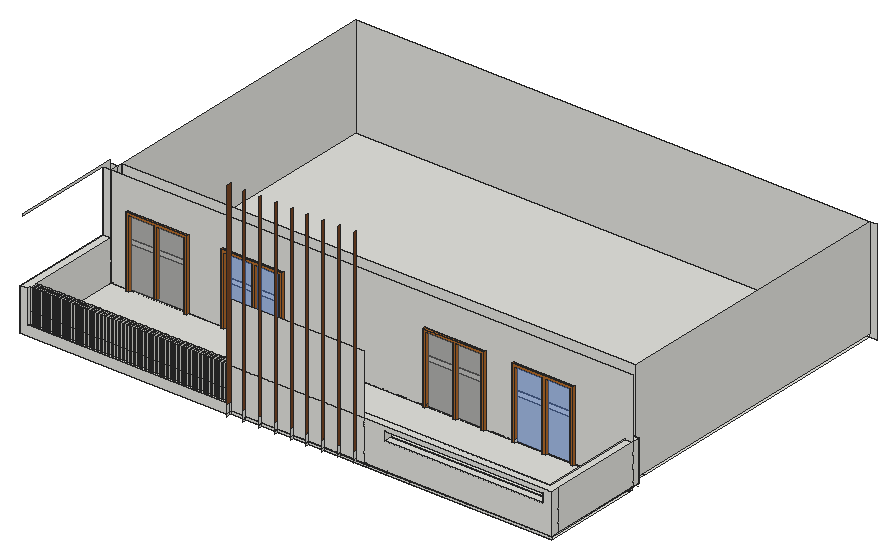
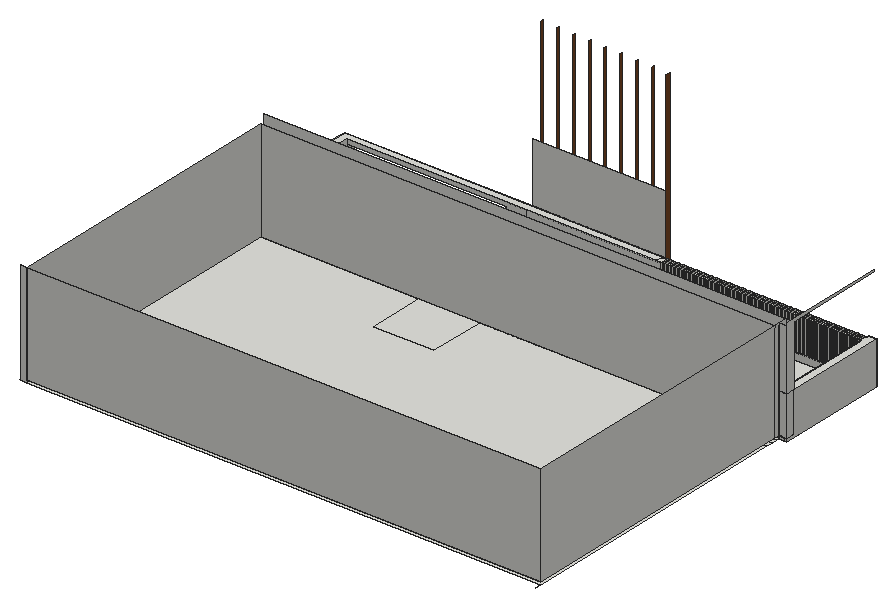
# SketchUp Ruby script. Lengths in inches.
U = 1.inch
M = Sketchup.active_model
def pt(a) = Geom::Point3d.new(a.map { |v| v * U })
def face(e, loops, mat)
  f = e.add_face(loops[0].map { |a| pt(a) })
  loops[1..].each { |l| e.add_face(l.map { |a| pt(a) }).erase! }
  f.material = f.back_material = mat if mat
  f
end
# faces: each face lists its corners as indices into pts; further lists are holes
def faces(e, pts, list, mat = nil) = list.each { |f| face(e, (f[0].is_a?(Array) ? f : [f]).map { |l| l.map { |i| pts[i] } }, mat) }
# xy, xz, yz: faces in a plane at the given z, y or x. An outline is a flat list of corners, or four numbers for a rectangle; further outlines are holes
def ring(l) = l.size == 4 ? [[l[0], l[1]], [l[2], l[1]], [l[2], l[3]], [l[0], l[3]]] : l.each_slice(2).to_a
def flat(e, list, mat, &to3) = list.each { |f| face(e, (f[0].is_a?(Array) ? f : [f]).map { |l| ring(l).map { |u, v| to3.(u, v) } }, mat) }
def xy(e, z, list, mat = nil) = flat(e, list, mat) { |x, y| [x, y, z] }
def xz(e, y, list, mat = nil) = flat(e, list, mat) { |x, z| [x, y, z] }
def yz(e, x, list, mat = nil) = flat(e, list, mat) { |y, z| [x, y, z] }
def lines(e, pts, list) = list.each { |a, b| e.add_line(pt(pts[a]), pt(pts[b])) }
# prism: a flat outline (further loops are holes) pulled along v
def prism(e, loops, v, mat = nil)
  f = face(e, loops, mat); d = Geom::Vector3d.new(v.map { |x| x * U })
  f.pushpull(f.normal.samedirection?(d) ? d.length : -d.length)
end
def box(e, o, s, mat = nil) = prism(e, [[o, [o[0] + s[0], o[1], o[2]], [o[0] + s[0], o[1] + s[1], o[2]], [o[0], o[1] + s[1], o[2]]]], [0, 0, s[2]], mat)
def at(x, y, z, deg = 0) = Geom::Transformation.translation(pt([x, y, z])) * Geom::Transformation.rotation(ORIGIN, Z_AXIS, deg.degrees)
def axes(o, x, y, z) = Geom::Transformation.new([*x, 0, *y, 0, *z, 0, *pt(o).to_a, 1])
def part(name) = M.definitions.add(name)
# library, detail: a bought-in or finely detailed component or shape, given as its bounding box
def library(name, o, s) = part(name).tap { |d| box(d.entities, o, s) }
def detail(e, o, s) = box(e.add_group.entities, o, s)
def put(e, d, t, mat = nil) = e.add_instance(d, t).tap { |i| i.material = mat if mat }
def group(e, t, mat = nil) = e.add_group.tap { |g| g.transformation = t; g.material = mat if mat }.entities
root = M.entities
M.materials.add("[Translucent Glass Blue]").color = [100, 149, 237]
M.materials["[Translucent Glass Blue]"].alpha = 0.5
M.materials.add("[Translucent Glass Gray]").color = [128, 128, 128]
M.materials["[Translucent Glass Gray]"].alpha = 0.5
M.materials.add("[Wood Bamboo]").color = [177, 105, 43]
M.materials.add("[Wood Veneer 01]").color = [120, 70, 37]
xy(root,243,[[0,3,9,15],[9,3,9,121.57,630,121.57,630,6,248.625,6,248.625,3],[0,15,9,121.57],[0,121.57,9,125.58],[9,121.57,621,125.58],
  [0,125.58,9,125.83],[9,125.58,621,125.83],[621,125.58,628.8125,125.83],[628.8125,125.58,629.5625,125.83],[629.5625,125.58,629.8125,125.83],
  [0,125.83,9,135.01],[9,125.83,621,135.01],[0,135.01,9,136.3125],[9,135.01,621,139.19],[9,139.19,621,146.07],
  [9,146.07,621,155.08],[9,155.08,621,490.375]])
xy(root,246,[[29.88,123.125,32.88,126.125],[98.88,123.125,101.88,126.125],[143,123.125,146,126.125],[212,123.125,215,126.125],[383.2,123.125,385.87,126.125],
  [419.2,123.125,422.35,126.125],[452.18,123.125,455.2,126.125],[489.07,123.125,492.05,126.125],[525.07,123.125,528.74,126.125],[558.54,123.125,561.07,126.125],
  [621,125.58,628.8125,126.125],[628.8125,125.58,629.5625,126.125],[629.5625,125.58,629.8125,126.125],[0,126.125,9,135.0625],[9,126.125,360.67,135.0625],
  [360.67,126.125,432.67,135.0625],[432.67,126.125,620.5,135.0625],[620.5,126.125,621,135.0625],[621,126.125,628.8125,135.0625],[628.8125,126.125,630,135.0625],
  [0,135.0625,9,136.3125],[9,135.0625,360.67,136.3125],[360.67,135.0625,432.67,136.3125],[432.67,135.0625,620.5,136.3125],[620.5,135.0625,621,136.3125],
  [621,135.0625,628.8125,136.3125],[628.8125,135.0625,630,136.3125],[9,136.3125,360.67,142.3125],[360.67,136.3125,432.67,142.3125],[432.67,136.3125,621,142.3125],
  [9,142.3125,360.67,142.3125,360.67,210.125,432.67,210.125,432.67,142.3125,621,142.3125,621,490.375,9,490.375],[360.67,142.3125,432.67,210.125]])
xy(root,246.0625,[[9,15,621,127.3125]])
xy(root,249,[[63.3125,123.125,65.88,126.125],[179,123.125,182.42,126.125]])
xy(root,254.79,[[9,3,248.625,3,248.625,6,246.32,6,246.32,15,244.25,15,244.25,6,241.94,6,241.94,15,239.875,15,239.875,6,237.57,6,237.57,15,235.5,15,235.5,6,233.19,6,233.19,15,231.125,15,231.125,6,228.82,6,228.82,15,226.75,15,226.75,6,224.44,6,224.44,15,222.375,15,222.375,6,220.07,6,220.07,15,218,15,218,6,215.69,6,215.69,15,213.625,15,213.625,6,211.32,6,211.32,15,209.25,15,209.25,6,206.94,6,206.94,15,204.875,15,204.875,6,202.57,6,202.57,15,200.5,15,200.5,6,198.19,6,198.19,15,196.125,15,196.125,6,193.82,6,193.82,15,191.75,15,191.75,6,189.44,6,189.44,15,187.375,15,187.375,6,185.07,6,185.07,15,183,15,183,6,180.69,6,180.69,15,178.625,15,178.625,6,176.32,6,176.32,15,174.25,15,174.25,6,171.94,6,171.94,15,169.875,15,169.875,6,167.57,6,167.57,15,165.5,15,165.5,6,163.19,6,163.19,15,161.125,15,161.125,6,158.82,6,158.82,15,156.75,15,156.75,6,154.44,6,154.44,15,152.375,15,152.375,6,150.07,6,150.07,15,148,15,148,6,145.69,6,145.69,15,143.625,15,143.625,6,141.32,6,141.32,15,139.25,15,139.25,6,136.94,6,136.94,15,134.875,15,134.875,6,132.57,6,132.57,15,130.5,15,130.5,6,128.19,6,128.19,15,126.125,15,126.125,6,123.82,6,123.82,15,121.75,15,121.75,6,119.44,6,119.44,15,117.375,15,117.375,6,115.07,6,115.07,15,113,15,113,6,110.69,6,110.69,15,108.625,15,108.625,6,106.32,6,106.32,15,104.25,15,104.25,6,101.94,6,101.94,15,99.875,15,99.875,6,97.57,6,97.57,15,95.5,15,95.5,6,93.19,6,93.19,15,91.125,15,91.125,6,88.82,6,88.82,15,86.75,15,86.75,6,84.44,6,84.44,15,82.375,15,82.375,6,80.07,6,80.07,15,78,15,78,6,75.69,6,75.69,15,73.625,15,73.625,6,71.32,6,71.32,15,69.6875,15,69.6875,6,67.38,6,67.38,15,65.75,15,65.75,6,63.44,6,63.44,15,61.8125,15,61.8125,6,59.51,6,59.51,15,57.875,15,57.875,6,55.57,6,55.57,15,53.9375,15,53.9375,6,51.63,6,51.63,15,50,15,50,6,47.69,6,47.69,15,46.0625,15,46.0625,6,43.76,6,43.76,15,42.125,15,42.125,6,39.82,6,39.82,15,38.1875,15,38.1875,6,35.88,6,35.88,15,34.25,15,34.25,6,31.94,6,31.94,15,30.3125,15,30.3125,6,28.01,6,28.01,15,26.375,15,26.375,6,24.07,6,24.07,15,22.4375,15,22.4375,6,20.13,6,20.13,15,18.5,15,18.5,6,16.19,6,16.19,15,14.5625,15,14.5625,6,12.26,6,12.26,15,10.625,15,10.625,6,9,6]])
xy(root,278.79,[[431.43,6,619.93,15]])
xy(root,289.1,[[431.43,6,619.93,15]])
xy(root,294.0625,[[0,3,9,3,9,6,10.625,6,10.625,15,9,15,9,127.3125,621,127.3125,621,15,255.92,15,248.625,6,630,6,630,136.3125,0,136.3125],[12.26,6,14.5625,15],[16.19,6,18.5,15],[20.13,6,22.4375,15],[24.07,6,26.375,15],
  [28.01,6,30.3125,15],[31.94,6,34.25,15],[35.88,6,38.1875,15],[39.82,6,42.125,15],[43.76,6,46.0625,15],
  [47.69,6,50,15],[51.63,6,53.9375,15],[55.57,6,57.875,15],[59.51,6,61.8125,15],[63.44,6,65.75,15],
  [67.38,6,69.6875,15],[71.32,6,73.625,15],[75.69,6,78,15],[80.07,6,82.375,15],[84.44,6,86.75,15],
  [88.82,6,91.125,15],[93.19,6,95.5,15],[97.57,6,99.875,15],[101.94,6,104.25,15],[106.32,6,108.625,15],
  [110.69,6,113,15],[115.07,6,117.375,15],[119.44,6,121.75,15],[123.82,6,126.125,15],[128.19,6,130.5,15],
  [132.57,6,134.875,15],[136.94,6,139.25,15],[141.32,6,143.625,15],[145.69,6,148,15],[150.07,6,152.375,15],
  [154.44,6,156.75,15],[158.82,6,161.125,15],[163.19,6,165.5,15],[167.57,6,169.875,15],[171.94,6,174.25,15],
  [176.32,6,178.625,15],[180.69,6,183,15],[185.07,6,187.375,15],[189.44,6,191.75,15],[193.82,6,196.125,15],
  [198.19,6,200.5,15],[202.57,6,204.875,15],[206.94,6,209.25,15],[211.32,6,213.625,15],[215.69,6,218,15],
  [220.07,6,222.375,15],[224.44,6,226.75,15],[228.82,6,231.125,15],[233.19,6,235.5,15],[237.57,6,239.875,15],
  [241.94,6,244.25,15],[246.32,6,248.625,6,255.92,15,246.32,15]])
xy(root,327,[[32.88,123.125,63.3125,126.125],[65.88,123.125,98.88,126.125],[146,123.125,179,126.125],[182.42,123.125,212,126.125],[386.2,123.125,419.2,126.125],
  [422.35,123.125,452.2,126.125],[492.07,123.125,525.07,126.125],[528.74,123.125,558.07,126.125]],"[Wood Bamboo]")
xy(root,330,[[29.88,123.125,101.88,126.125],[143,123.125,215,126.125],[383.2,123.125,455.2,126.125],[489.07,123.125,561.07,126.125]],"[Wood Bamboo]")
xz(root,3,[[0,243,248.625,243,248.625,254.79,9,254.79,9,294.0625,0,294.0625]])
xz(root,6,[[248.625,243,406.875,245.8125],[406.875,243,630,245.8125],[248.625,245.8125,406.875,246],[406.875,245.8125,630,246],[248.625,246,406.875,246.0625],
  [406.875,246,630,246.0625],[248.625,246.0625,406.875,294.0625],[[406.875,246.0625,630,294.0625],[431.43,278.79,619.93,289.1]],[8.32,254.79,9,294.0625],[9,254.79,10.625,294.0625],
  [12.26,254.79,14.5625,294.0625],[16.19,254.79,18.5,294.0625],[20.13,254.79,22.4375,294.0625],[24.07,254.79,26.375,294.0625],[28.01,254.79,30.3125,294.0625],
  [31.94,254.79,34.25,294.0625],[35.88,254.79,38.1875,294.0625],[39.82,254.79,42.125,294.0625],[43.76,254.79,46.0625,294.0625],[47.69,254.79,50,294.0625],
  [51.63,254.79,53.9375,294.0625],[55.57,254.79,57.875,294.0625],[59.51,254.79,61.8125,294.0625],[63.44,254.79,65.75,294.0625],[67.38,254.79,69.6875,294.0625],
  [71.32,254.79,73.625,294.0625],[75.69,254.79,78,294.0625],[80.07,254.79,82.375,294.0625],[84.44,254.79,86.75,294.0625],[88.82,254.79,91.125,294.0625],
  [93.19,254.79,95.5,294.0625],[97.57,254.79,99.875,294.0625],[101.94,254.79,104.25,294.0625],[106.32,254.79,108.625,294.0625],[110.69,254.79,113,294.0625],
  [115.07,254.79,117.375,294.0625],[119.44,254.79,121.75,294.0625],[123.82,254.79,126.125,294.0625],[128.19,254.79,130.5,294.0625],[132.57,254.79,134.875,294.0625],
  [136.94,254.79,139.25,294.0625],[141.32,254.79,143.625,294.0625],[145.69,254.79,148,294.0625],[150.07,254.79,152.375,294.0625],[154.44,254.79,156.75,294.0625],
  [158.82,254.79,161.125,294.0625],[163.19,254.79,165.5,294.0625],[167.57,254.79,169.875,294.0625],[171.94,254.79,174.25,294.0625],[176.32,254.79,178.625,294.0625],
  [180.69,254.79,183,294.0625],[185.07,254.79,187.375,294.0625],[189.44,254.79,191.75,294.0625],[193.82,254.79,196.125,294.0625],[198.19,254.79,200.5,294.0625],
  [202.57,254.79,204.875,294.0625],[206.94,254.79,209.25,294.0625],[211.32,254.79,213.625,294.0625],[215.69,254.79,218,294.0625],[220.07,254.79,222.375,294.0625],
  [224.44,254.79,226.75,294.0625],[228.82,254.79,231.125,294.0625],[233.19,254.79,235.5,294.0625],[237.57,254.79,239.875,294.0625],[241.94,254.79,244.25,294.0625],
  [246.32,254.79,248.625,294.0625],[248.625,294.0625,406.875,366]])
xz(root,15,[[9,246.0625,9,294.0625,10.625,294.0625,10.625,254.79,12.26,254.79,12.26,294.0625,14.5625,294.0625,14.5625,254.79,16.19,254.79,16.19,294.0625,18.5,294.0625,18.5,254.79,20.13,254.79,20.13,294.0625,22.4375,294.0625,22.4375,254.79,24.07,254.79,24.07,294.0625,26.375,294.0625,26.375,254.79,28.01,254.79,28.01,294.0625,30.3125,294.0625,30.3125,254.79,31.94,254.79,31.94,294.0625,34.25,294.0625,34.25,254.79,35.88,254.79,35.88,294.0625,38.1875,294.0625,38.1875,254.79,39.82,254.79,39.82,294.0625,42.125,294.0625,42.125,254.79,43.76,254.79,43.76,294.0625,46.0625,294.0625,46.0625,254.79,47.69,254.79,47.69,294.0625,50,294.0625,50,254.79,51.63,254.79,51.63,294.0625,53.9375,294.0625,53.9375,254.79,55.57,254.79,55.57,294.0625,57.875,294.0625,57.875,254.79,59.51,254.79,59.51,294.0625,61.8125,294.0625,61.8125,254.79,63.44,254.79,63.44,294.0625,65.75,294.0625,65.75,254.79,67.38,254.79,67.38,294.0625,69.6875,294.0625,69.6875,254.79,71.32,254.79,71.32,294.0625,73.625,294.0625,73.625,254.79,75.69,254.79,75.69,294.0625,78,294.0625,78,254.79,80.07,254.79,80.07,294.0625,82.375,294.0625,82.375,254.79,84.44,254.79,84.44,294.0625,86.75,294.0625,86.75,254.79,88.82,254.79,88.82,294.0625,91.125,294.0625,91.125,254.79,93.19,254.79,93.19,294.0625,95.5,294.0625,95.5,254.79,97.57,254.79,97.57,294.0625,99.875,294.0625,99.875,254.79,101.94,254.79,101.94,294.0625,104.25,294.0625,104.25,254.79,106.32,254.79,106.32,294.0625,108.625,294.0625,108.625,254.79,110.69,254.79,110.69,294.0625,113,294.0625,113,254.79,115.07,254.79,115.07,294.0625,117.375,294.0625,117.375,254.79,119.44,254.79,119.44,294.0625,121.75,294.0625,121.75,254.79,123.82,254.79,123.82,294.0625,126.125,294.0625,126.125,254.79,128.19,254.79,128.19,294.0625,130.5,294.0625,130.5,254.79,132.57,254.79,132.57,294.0625,134.875,294.0625,134.875,254.79,136.94,254.79,136.94,294.0625,139.25,294.0625,139.25,254.79,141.32,254.79,141.32,294.0625,143.625,294.0625,143.625,254.79,145.69,254.79,145.69,294.0625,148,294.0625,148,254.79,150.07,254.79,150.07,294.0625,152.375,294.0625,152.375,254.79,154.44,254.79,154.44,294.0625,156.75,294.0625,156.75,254.79,158.82,254.79,158.82,294.0625,161.125,294.0625,161.125,254.79,163.19,254.79,163.19,294.0625,165.5,294.0625,165.5,254.79,167.57,254.79,167.57,294.0625,169.875,294.0625,169.875,254.79,171.94,254.79,171.94,294.0625,174.25,294.0625,174.25,254.79,176.32,254.79,176.32,294.0625,178.625,294.0625,178.625,254.79,180.69,254.79,180.69,294.0625,183,294.0625,183,254.79,185.07,254.79,185.07,294.0625,187.375,294.0625,187.375,254.79,189.44,254.79,189.44,294.0625,191.75,294.0625,191.75,254.79,193.82,254.79,193.82,294.0625,196.125,294.0625,196.125,254.79,198.19,254.79,198.19,294.0625,200.5,294.0625,200.5,254.79,202.57,254.79,202.57,294.0625,204.875,294.0625,204.875,254.79,206.94,254.79,206.94,294.0625,209.25,294.0625,209.25,254.79,211.32,254.79,211.32,294.0625,213.625,294.0625,213.625,254.79,215.69,254.79,215.69,294.0625,218,294.0625,218,254.79,220.07,254.79,220.07,294.0625,222.375,294.0625,222.375,254.79,224.44,254.79,224.44,294.0625,226.75,294.0625,226.75,254.79,228.82,254.79,228.82,294.0625,231.125,294.0625,231.125,254.79,233.19,254.79,233.19,294.0625,235.5,294.0625,235.5,254.79,237.57,254.79,237.57,294.0625,239.875,294.0625,239.875,254.79,241.94,254.79,241.94,294.0625,244.25,294.0625,244.25,254.79,246.32,254.79,246.32,294.0625,248.625,294.0625,248.625,246.0625],[248.625,246.0625,406.875,294.0625],[[406.875,246.0625,621,294.0625],[431.43,278.79,619.93,289.1]]])
xz(root,123.125,[[29.88,246,32.88,246,32.88,327,63.3125,327,63.3125,249,65.88,249,65.88,327,98.88,327,98.88,246,101.88,246,101.88,330,29.88,330],[143,246,146,246,146,327,179,327,179,249,182.42,249,182.42,327,212,327,212,246,215,246,215,330,143,330],[383.2,246,385.87,246,386.2,249,386.2,327,419.2,327,419.2,246,422.35,246,422.35,327,452.2,327,452.2,249,452.18,246,455.2,246,455.2,330,383.2,330],[489.07,246,492.05,246,492.07,249,492.07,327,525.07,327,525.07,246,528.74,246,528.74,327,558.07,327,558.07,249,558.54,246,561.07,246,561.07,330,489.07,330]],"[Wood Bamboo]")
xz(root,125.58,[[621,243,628.8125,245.8125],[628.8125,243,629.5625,245.8125],[629.5625,243,629.8125,245.8125],[621,245.8125,628.8125,246],[628.8125,245.8125,629.5625,246],
  [629.5625,245.8125,629.8125,246]])
xz(root,126.125,[[9,245.8125,32.88,246],[32.88,245.8125,98.88,246],[98.88,245.8125,630,246],[0,246,9,366.375],[9,246,29.88,246,29.88,330,101.88,330,101.88,246,143,246,143,330,215,330,215,246,383.2,246,383.2,330,455.2,330,455.2,246,489.07,246,489.07,330,561.07,330,561.07,246,630,246,630,366.375,9,366.375],
  [29.88,246,29.88,330,101.88,330,101.88,246,98.88,246,98.88,327,65.88,327,65.88,249,63.3125,249,63.3125,327,32.88,327,32.88,246],[143,246,143,330,215,330,215,246,212,246,212,327,182.42,327,182.42,249,179,249,179,327,146,327,146,246],[383.2,246,383.2,330,455.2,330,455.2,246,452.18,246,452.2,249,452.2,327,422.35,327,422.35,246,419.2,246,419.2,327,386.2,327,386.2,249,385.87,246],[489.07,246,489.07,330,561.07,330,561.07,246,558.54,246,558.07,249,558.07,327,528.74,327,528.74,246,525.07,246,525.07,327,492.07,327,492.07,249,492.05,246]])
xz(root,126.125,[[146,246,212,246,212,327,182.42,327,182.42,249,179,249,179,327,146,327],[492.05,246,525.07,246,525.07,327,492.07,327,492.07,249],[528.74,246,558.54,246,558.07,249,558.07,327,528.74,327]],"[Translucent Glass Blue]")
xz(root,126.125,[[32.88,246,98.88,246,98.88,327,65.88,327,65.88,249,63.3125,249,63.3125,327,32.88,327],[385.87,246,419.2,246,419.2,327,386.2,327,386.2,249],[422.35,246,452.18,246,452.2,249,452.2,327,422.35,327]],"[Translucent Glass Gray]")
xz(root,127.3125,[[9,246.0625,621,294.0625]])
xz(root,136.3125,[[0,243,9,246],[0,246,9,246.0625],[9,246,630,246.0625],[0,246.0625,9,294.0625],[9,246.0625,630,294.0625],
  [0,294.0625,9,366]])
xz(root,142.3125,[[9,246,621,366]])
xz(root,490.375,[[620.75,243,628.8125,243,628.8125,366,621,366,621,246,620.75,246],[9,246,620.75,366],[620.75,246,621,366]])
yz(root,0,[[3,243,3,294.0625,126.125,294.0625,126.125,246,136.3125,246,136.3125,243],[126.125,246,136.3125,246.0625],[126.125,246.0625,136.3125,294.0625],[126.125,294.0625,126.125,366.375,6,366.375,6,369,136.3125,369,136.3125,294.0625]])
yz(root,9,[[121.57,243,136.3125,243,136.3125,246,126.125,246,126.125,245.8125,121.57,245.8125],[121.57,245.8125,126.125,246],[126.125,246,136.3125,246,136.3125,366,126.125,366,126.125,294.0625,127.3125,294.0625,127.3125,246.0625,126.125,246.0625],[136.3125,246,142.3125,366],[142.3125,246,490.375,366],
  [15,246.0625,126.125,294.0625],[126.125,246.0625,127.3125,294.0625],[3,254.79,6,294.0625]])
yz(root,10.625,[[6,254.79,15,267.71],[6,267.71,15,294.0625]])
yz(root,12.26,[[6,254.79,15,294.0625]])
yz(root,14.5625,[[6,254.79,15,267.71],[6,267.71,15,294.0625]])
yz(root,16.19,[[6,254.79,15,294.0625]])
yz(root,18.5,[[6,254.79,15,267.71],[6,267.71,15,294.0625]])
yz(root,20.13,[[6,254.79,15,294.0625]])
yz(root,22.4375,[[6,254.79,15,267.71],[6,267.71,15,294.0625]])
yz(root,24.07,[[6,254.79,15,294.0625]])
yz(root,26.375,[[6,254.79,15,267.71],[6,267.71,15,294.0625]])
yz(root,28.01,[[6,254.79,15,294.0625]])
yz(root,29.88,[[123.125,246,126.125,330]],"[Wood Bamboo]")
yz(root,30.3125,[[6,254.79,15,267.71],[6,267.71,15,294.0625]])
yz(root,31.94,[[6,254.79,15,294.0625]])
yz(root,32.88,[[123.125,246,126.125,327]],"[Wood Bamboo]")
yz(root,34.25,[[6,254.79,15,267.71],[6,267.71,15,294.0625]])
yz(root,35.88,[[6,254.79,15,294.0625]])
yz(root,38.1875,[[6,254.79,15,267.71],[6,267.71,15,294.0625]])
yz(root,39.82,[[6,254.79,15,294.0625]])
yz(root,42.125,[[6,254.79,15,267.71],[6,267.71,15,294.0625]])
yz(root,43.76,[[6,254.79,15,294.0625]])
yz(root,46.0625,[[6,254.79,15,267.71],[6,267.71,15,294.0625]])
yz(root,47.69,[[6,254.79,15,294.0625]])
yz(root,50,[[6,254.79,15,267.71],[6,267.71,15,294.0625]])
yz(root,51.63,[[6,254.79,15,294.0625]])
yz(root,53.9375,[[6,254.79,15,267.71],[6,267.71,15,294.0625]])
yz(root,55.57,[[6,254.79,15,294.0625]])
yz(root,57.875,[[6,254.79,15,267.71],[6,267.71,15,294.0625]])
yz(root,59.51,[[6,254.79,15,294.0625]])
yz(root,61.8125,[[6,254.79,15,267.71],[6,267.71,15,294.0625]])
yz(root,63.3125,[[123.125,249,126.125,327]],"[Wood Bamboo]")
yz(root,63.44,[[6,254.79,15,294.0625]])
yz(root,65.75,[[6,254.79,15,267.71],[6,267.71,15,294.0625]])
yz(root,65.88,[[123.125,249,126.125,327]],"[Wood Bamboo]")
yz(root,67.38,[[6,254.79,15,294.0625]])
yz(root,69.6875,[[6,254.79,15,267.71],[6,267.71,15,294.0625]])
yz(root,71.32,[[6,254.79,15,294.0625]])
yz(root,73.625,[[6,254.79,15,267.71],[6,267.71,15,294.0625]])
yz(root,75.69,[[6,254.79,15,294.0625]])
yz(root,78,[[6,254.79,15,267.71],[6,267.71,15,294.0625]])
yz(root,80.07,[[6,254.79,15,294.0625]])
yz(root,82.375,[[6,254.79,15,267.71],[6,267.71,15,294.0625]])
yz(root,84.44,[[6,254.79,15,294.0625]])
yz(root,86.75,[[6,254.79,15,267.71],[6,267.71,15,294.0625]])
yz(root,88.82,[[6,254.79,15,294.0625]])
yz(root,91.125,[[6,254.79,15,267.71],[6,267.71,15,294.0625]])
yz(root,93.19,[[6,254.79,15,294.0625]])
yz(root,95.5,[[6,254.79,15,267.71],[6,267.71,15,294.0625]])
yz(root,97.57,[[6,254.79,15,294.0625]])
yz(root,98.88,[[123.125,246,126.125,327]],"[Wood Bamboo]")
yz(root,99.875,[[6,254.79,15,267.71],[6,267.71,15,294.0625]])
yz(root,101.88,[[123.125,246,126.125,330]],"[Wood Bamboo]")
yz(root,101.94,[[6,254.79,15,294.0625]])
yz(root,104.25,[[6,254.79,15,267.71],[6,267.71,15,294.0625]])
yz(root,106.32,[[6,254.79,15,294.0625]])
yz(root,108.625,[[6,254.79,15,267.71],[6,267.71,15,294.0625]])
yz(root,110.69,[[6,254.79,15,294.0625]])
yz(root,113,[[6,254.79,15,267.71],[6,267.71,15,294.0625]])
yz(root,115.07,[[6,254.79,15,294.0625]])
yz(root,117.375,[[6,254.79,15,267.71],[6,267.71,15,294.0625]])
yz(root,119.44,[[6,254.79,15,294.0625]])
yz(root,121.75,[[6,254.79,15,267.71],[6,267.71,15,294.0625]])
yz(root,123.82,[[6,254.79,15,294.0625]])
yz(root,126.125,[[6,254.79,15,267.71],[6,267.71,15,294.0625]])
yz(root,128.19,[[6,254.79,15,294.0625]])
yz(root,130.5,[[6,254.79,15,267.71],[6,267.71,15,294.0625]])
yz(root,132.57,[[6,254.79,15,294.0625]])
yz(root,134.875,[[6,254.79,15,267.71],[6,267.71,15,294.0625]])
yz(root,136.94,[[6,254.79,15,294.0625]])
yz(root,139.25,[[6,254.79,15,267.71],[6,267.71,15,294.0625]])
yz(root,141.32,[[6,254.79,15,294.0625]])
yz(root,143,[[123.125,246,126.125,330]],"[Wood Bamboo]")
yz(root,143.625,[[6,254.79,15,267.71],[6,267.71,15,294.0625]])
yz(root,145.69,[[6,254.79,15,294.0625]])
yz(root,146,[[123.125,246,126.125,327]],"[Wood Bamboo]")
yz(root,148,[[6,254.79,15,267.71],[6,267.71,15,294.0625]])
yz(root,150.07,[[6,254.79,15,294.0625]])
yz(root,152.375,[[6,254.79,15,267.71],[6,267.71,15,294.0625]])
yz(root,154.44,[[6,254.79,15,294.0625]])
yz(root,156.75,[[6,254.79,15,267.71],[6,267.71,15,294.0625]])
yz(root,158.82,[[6,254.79,15,294.0625]])
yz(root,161.125,[[6,254.79,15,267.71],[6,267.71,15,294.0625]])
yz(root,163.19,[[6,254.79,15,294.0625]])
yz(root,165.5,[[6,254.79,15,267.71],[6,267.71,15,294.0625]])
yz(root,167.57,[[6,254.79,15,294.0625]])
yz(root,169.875,[[6,254.79,15,267.71],[6,267.71,15,294.0625]])
yz(root,171.94,[[6,254.79,15,294.0625]])
yz(root,174.25,[[6,254.79,15,267.71],[6,267.71,15,294.0625]])
yz(root,176.32,[[6,254.79,15,294.0625]])
yz(root,178.625,[[6,254.79,15,267.71],[6,267.71,15,294.0625]])
yz(root,179,[[123.125,249,126.125,327]],"[Wood Bamboo]")
yz(root,180.69,[[6,254.79,15,294.0625]])
yz(root,182.42,[[123.125,249,126.125,327]],"[Wood Bamboo]")
yz(root,183,[[6,254.79,15,267.71],[6,267.71,15,294.0625]])
yz(root,185.07,[[6,254.79,15,294.0625]])
yz(root,187.375,[[6,254.79,15,267.71],[6,267.71,15,294.0625]])
yz(root,189.44,[[6,254.79,15,294.0625]])
yz(root,191.75,[[6,254.79,15,267.71],[6,267.71,15,294.0625]])
yz(root,193.82,[[6,254.79,15,294.0625]])
yz(root,196.125,[[6,254.79,15,267.71],[6,267.71,15,294.0625]])
yz(root,198.19,[[6,254.79,15,294.0625]])
yz(root,200.5,[[6,254.79,15,267.71],[6,267.71,15,294.0625]])
yz(root,202.57,[[6,254.79,15,294.0625]])
yz(root,204.875,[[6,254.79,15,267.71],[6,267.71,15,294.0625]])
yz(root,206.94,[[6,254.79,15,294.0625]])
yz(root,209.25,[[6,254.79,15,267.71],[6,267.71,15,294.0625]])
yz(root,211.32,[[6,254.79,15,294.0625]])
yz(root,212,[[123.125,246,126.125,327]],"[Wood Bamboo]")
yz(root,213.625,[[6,254.79,15,267.71],[6,267.71,15,294.0625]])
yz(root,215,[[123.125,246,126.125,330]],"[Wood Bamboo]")
yz(root,215.69,[[6,254.79,15,294.0625]])
yz(root,218,[[6,254.79,15,267.71],[6,267.71,15,294.0625]])
yz(root,220.07,[[6,254.79,15,294.0625]])
yz(root,222.375,[[6,254.79,15,267.71],[6,267.71,15,294.0625]])
yz(root,224.44,[[6,254.79,15,294.0625]])
yz(root,226.75,[[6,254.79,15,267.71],[6,267.71,15,294.0625]])
yz(root,228.82,[[6,254.79,15,294.0625]])
yz(root,231.125,[[6,254.79,15,267.71],[6,267.71,15,294.0625]])
yz(root,233.19,[[6,254.79,15,294.0625]])
yz(root,235.5,[[6,254.79,15,267.71],[6,267.71,15,294.0625]])
yz(root,237.57,[[6,254.79,15,294.0625]])
yz(root,239.875,[[6,254.79,15,267.71],[6,267.71,15,294.0625]])
yz(root,241.94,[[6,254.79,15,294.0625]])
yz(root,244.25,[[6,254.79,15,267.71],[6,267.71,15,294.0625]])
yz(root,246.32,[[6,254.79,15,294.0625]])
yz(root,248.625,[[0,243,3,245.8125],[3,243,6,245.8125],[0,245.8125,3,246],[3,245.8125,6,246],[0,246,3,246.0625],
  [3,246,6,246.0625],[0,246.0625,3,254.79],[3,246.0625,6,254.79]])
yz(root,248.625,[[0,254.79,6,489]],"[Wood Veneer 01]")
yz(root,267.4375,[[0,243.375,3,246.1875],[0,246.1875,3,246.375],[0,246.375,3,246.4375],[0,246.4375,3,255.16]])
yz(root,267.4375,[[0,255.16,3,489.375]],"[Wood Veneer 01]")
yz(root,286.25,[[0,243.75,3,246.5625],[0,246.5625,3,246.75],[0,246.75,3,246.8125],[0,246.8125,3,255.54]])
yz(root,286.25,[[0,255.54,3,489.75]],"[Wood Veneer 01]")
yz(root,305.06,[[0,244.125,3,246.9375],[0,246.9375,3,247.125],[0,247.125,3,247.1875],[0,247.1875,3,255.91]])
yz(root,305.06,[[0,255.91,3,490.125]],"[Wood Veneer 01]")
yz(root,323.87,[[0,244.5,3,247.3125],[0,247.3125,3,247.5],[0,247.5,3,247.5625],[0,247.5625,3,256.29]])
yz(root,323.87,[[0,256.29,3,490.5]],"[Wood Veneer 01]")
yz(root,342.68,[[0,244.875,3,247.6875],[0,247.6875,3,247.875],[0,247.875,3,247.9375],[0,247.9375,3,256.66]])
yz(root,342.68,[[0,256.66,3,490.875]],"[Wood Veneer 01]")
yz(root,361.49,[[0,245.25,3,248.0625],[0,248.0625,3,248.25],[0,248.25,3,248.3125],[0,248.3125,3,257.04]])
yz(root,361.49,[[0,257.04,3,491.25]],"[Wood Veneer 01]")
yz(root,380.31,[[0,245.625,3,248.4375],[0,248.4375,3,248.625],[0,248.625,3,248.6875],[0,248.6875,3,257.41]])
yz(root,380.31,[[0,257.41,3,491.625]],"[Wood Veneer 01]")
yz(root,383.2,[[123.125,246,126.125,330]],"[Wood Bamboo]")
yz(root,386.2,[[123.125,249,126.125,327]],"[Wood Bamboo]")
yz(root,399.12,[[0,246,3,248.8125],[0,248.8125,3,249],[0,249,3,249.0625],[0,249.0625,3,257.79]])
yz(root,399.12,[[0,257.79,3,492]],"[Wood Veneer 01]")
yz(root,419.2,[[123.125,246,126.125,327]],"[Wood Bamboo]")
yz(root,422.35,[[123.125,246,126.125,327]],"[Wood Bamboo]")
yz(root,431.43,[[6,278.79,15,289.1]])
yz(root,452.2,[[123.125,249,126.125,327]],"[Wood Bamboo]")
yz(root,455.2,[[123.125,246,126.125,330]],"[Wood Bamboo]")
yz(root,489.07,[[123.125,246,126.125,330]],"[Wood Bamboo]")
yz(root,492.07,[[123.125,249,126.125,327]],"[Wood Bamboo]")
yz(root,525.07,[[123.125,246,126.125,327]],"[Wood Bamboo]")
yz(root,528.74,[[123.125,246,126.125,327]],"[Wood Bamboo]")
yz(root,558.07,[[123.125,249,126.125,327]],"[Wood Bamboo]")
yz(root,561.07,[[123.125,246,126.125,330]],"[Wood Bamboo]")
yz(root,619.93,[[6,278.79,15,289.1]])
yz(root,621,[[142.3125,246,490.375,366],[15,246.0625,126.125,294.0625],[126.125,246.0625,127.3125,294.0625]])
yz(root,630,[[6,245.8125,14.4375,246],[14.4375,245.8125,125.58,246],[125.58,245.8125,126.125,246],[6,246,14.4375,246.0625],[14.4375,246,126.125,246.0625],
  [126.125,246,135.0625,246.0625],[135.0625,246,136.3125,246.0625],[6,246.0625,14.4375,294.0625],[14.4375,246.0625,126.125,294.0625],[126.125,246.0625,135.0625,294.0625],
  [135.0625,246.0625,136.3125,294.0625]])
p = [[385.87,126.125,246],[386.2,126.125,249],[386.2,123.125,249],[385.87,123.125,246],[452.2,126.125,249],[452.18,126.125,246],
  [452.18,123.125,246],[452.2,123.125,249],[492.05,126.125,246],[492.07,126.125,249],[492.07,123.125,249],[492.05,123.125,246],
  [558.07,126.125,249],[558.54,126.125,246],[558.54,123.125,246],[558.07,123.125,249],[9,490.375,243],[9,499.375,243],
  [628.8125,490.375,243],[630,490.375,243],[621,121.57,243],[621,121.57,245.8125],[629.8125,125.58,243],[630,125.58,243],
  [629.8125,125.58,245.8125],[630,125.58,245.8125],[621,135.01,243],[630,135.01,243],[6.6875,6,254.79],[4.38,6,254.79],
  [6.6875,6,267.71],[2.75,6,254.79],[0.44,6,254.79],[2.75,6,267.71],[417.93,3,249.4375],[417.93,3,249.375],
  [436.74,3,249.8125],[436.74,3,249.75],[436.74,3,249.5625]]
faces(root,p,[[0,1,2,3]],"[Wood Bamboo]")
faces(root,p,[[4,5,6,7],[8,9,10,11],[12,13,14,15]])
lines(root,p,[[16,17],[18,19],[20,21],[22,23],[24,25],[26,27],[28,29],[30,28],[31,32],[33,31],[34,35],[36,37],
  [37,38]])
